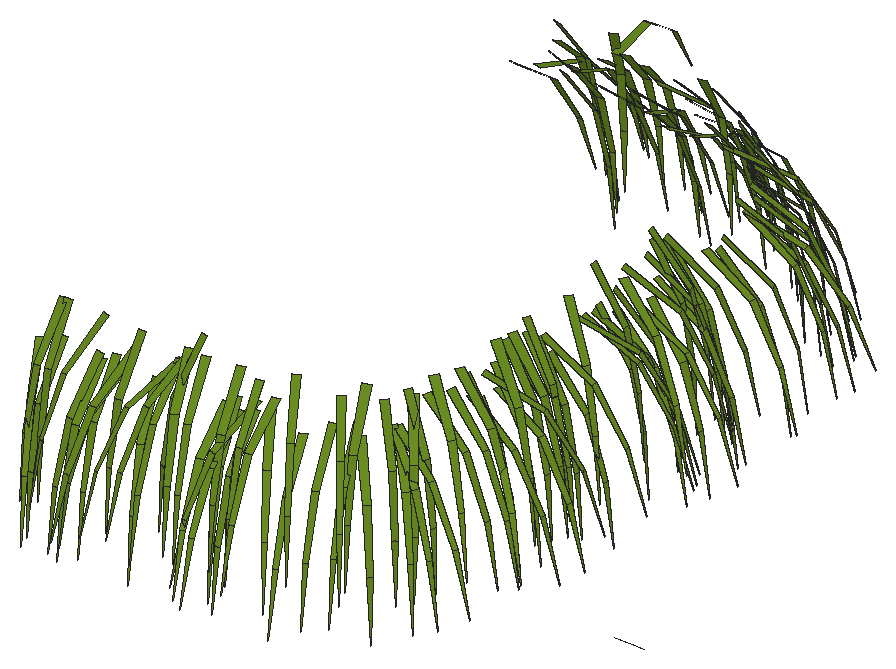
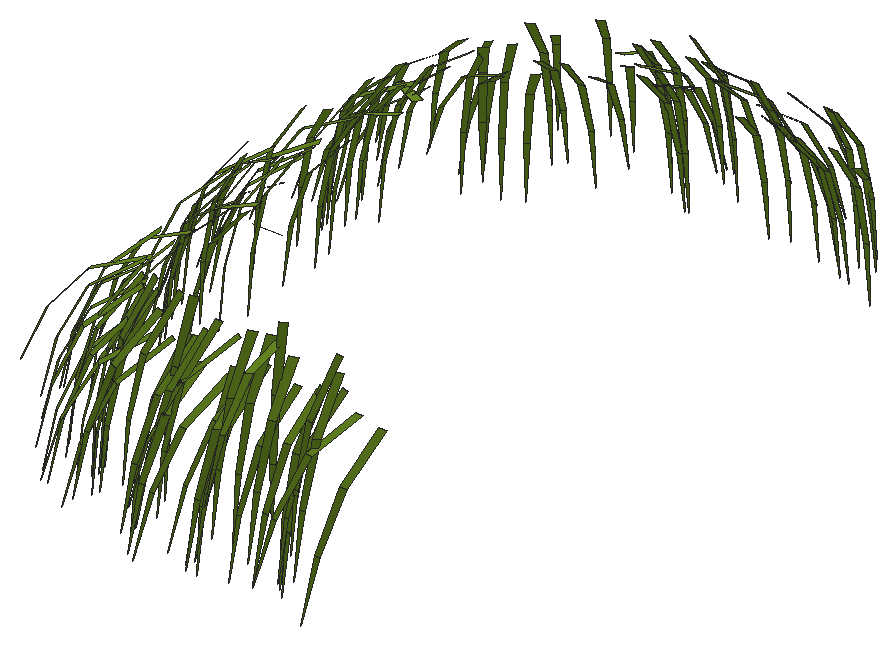
# SketchUp Ruby script. Lengths in inches.
U = 1.inch
M = Sketchup.active_model
def pt(a) = Geom::Point3d.new(a.map { |v| v * U })
def face(e, loops, mat)
  f = e.add_face(loops[0].map { |a| pt(a) })
  loops[1..].each { |l| e.add_face(l.map { |a| pt(a) }).erase! }
  f.material = f.back_material = mat if mat
  f
end
# faces: each face lists its corners as indices into pts; further lists are holes
def faces(e, pts, list, mat = nil) = list.each { |f| face(e, (f[0].is_a?(Array) ? f : [f]).map { |l| l.map { |i| pts[i] } }, mat) }
# xy, xz, yz: faces in a plane at the given z, y or x. An outline is a flat list of corners, or four numbers for a rectangle; further outlines are holes
def ring(l) = l.size == 4 ? [[l[0], l[1]], [l[2], l[1]], [l[2], l[3]], [l[0], l[3]]] : l.each_slice(2).to_a
def flat(e, list, mat, &to3) = list.each { |f| face(e, (f[0].is_a?(Array) ? f : [f]).map { |l| ring(l).map { |u, v| to3.(u, v) } }, mat) }
def xy(e, z, list, mat = nil) = flat(e, list, mat) { |x, y| [x, y, z] }
def xz(e, y, list, mat = nil) = flat(e, list, mat) { |x, z| [x, y, z] }
def yz(e, x, list, mat = nil) = flat(e, list, mat) { |y, z| [x, y, z] }
def lines(e, pts, list) = list.each { |a, b| e.add_line(pt(pts[a]), pt(pts[b])) }
# prism: a flat outline (further loops are holes) pulled along v
def prism(e, loops, v, mat = nil)
  f = face(e, loops, mat); d = Geom::Vector3d.new(v.map { |x| x * U })
  f.pushpull(f.normal.samedirection?(d) ? d.length : -d.length)
end
def box(e, o, s, mat = nil) = prism(e, [[o, [o[0] + s[0], o[1], o[2]], [o[0] + s[0], o[1] + s[1], o[2]], [o[0], o[1] + s[1], o[2]]]], [0, 0, s[2]], mat)
def at(x, y, z, deg = 0) = Geom::Transformation.translation(pt([x, y, z])) * Geom::Transformation.rotation(ORIGIN, Z_AXIS, deg.degrees)
def axes(o, x, y, z) = Geom::Transformation.new([*x, 0, *y, 0, *z, 0, *pt(o).to_a, 1])
def part(name) = M.definitions.add(name)
# library, detail: a bought-in or finely detailed component or shape, given as its bounding box
def library(name, o, s) = part(name).tap { |d| box(d.entities, o, s) }
def detail(e, o, s) = box(e.add_group.entities, o, s)
def put(e, d, t, mat = nil) = e.add_instance(d, t).tap { |i| i.material = mat if mat }
def group(e, t, mat = nil) = e.add_group.tap { |g| g.transformation = t; g.material = mat if mat }.entities
root = M.entities
M.materials.add("[0061_OliveDrab]").color = [107, 142, 35]
p = [[578.37,21.67,546.63],[578.33,21.46,546.63],[578.81,21.49,544.05],[575.9,5.78,546.69],[575.76,5.64,546.69],[576.08,5.46,544.09],
  [563.7,3.375,546.84],[563.51,3.36,546.84],[563.63,3,544.24],[561.71,4.01,546.8],[561.5,4.01,546.8],[561.6,3.83,544.18],
  [575.32,31.82,546.84],[575.47,31.67,546.84],[575.58,31.91,544.23],[563.21,3.55,546.9],[563,3.56,546.9],[563.08,3.2,544.3],
  [578.12,26.57,546.86],[578.17,26.37,546.86],[578.49,26.56,544.26],[574.38,32.14,546.9],[574.5625,32,546.9],[574.6,32.24,544.29],
  [578.36,16.1875,546.95],[578.35,15.98,546.95],[578.74,16.07,544.35],[576.49,31.86,546.99],[576.61,31.7,546.99],[576.97,32.09,544.42],
  [570.74,3.47,547.125],[570.52,3.4375,547.125],[570.68,3.08,544.53],[564.15,33.94,547.14],[564.36,33.9,547.14],[564.31,34.16,544.53],
  [566.98,3.28,547.16],[566.81,3.21,547.16],[567.07,2.8,544.58],[564.56,3.45,547.21],[564.375,3.42,547.21],[564.53,3.08,544.61],
  [562.19,3.09,547.22],[562.02,3,547.22],[562.43,2.45,544.68],[570.31,3.66,547.34],[570.13,3.61,547.34],[570.31,3.32,544.74],
  [574.0625,4.38,547.24],[573.88,4.32,547.24],[574.13,3.89,544.66],[577.73,19.19,547.37],[577.74,19,547.37],[577.94,19.11,544.75],
  [574.89,31.62,547.31],[575.04,31.49,547.31],[575.0625,31.67,544.69],[563.94,3.36,547.4],[563.73,3.44,547.4],[563.7,3.03,544.81],
  [578.58,22.99,547.34],[578.57,22.8,547.34],[579,22.875,544.75],[578.09,27.49,547.37],[578.17,27.33,547.37],[578.46,27.58,544.77],
  [567.45,34.65,547.39],[567.65,34.7,547.39],[567.41,35.2,544.82],[573.63,3.17,547.36],[573.45,3.1,547.36],[573.85,2.36,544.87],
  [577.32,6.34,547.47],[577.19,6.21,547.47],[577.78,5.77,544.95],[577.66,7.01,547.46],[577.57,6.84,547.46],[578.28,6.5625,544.95],
  [575.86,7.28,547.55],[575.74,7.12,547.55],[575.93,7.1,544.93],[577.81,15.24,547.53],[577.78,15.06,547.53],[578.05,15.11,544.92],
  [578.24,29.64,547.43],[578.3125,29.44,547.43],[578.88,29.75,544.88],[567.9,34.46,547.4375],[568.1,34.4,547.4375],[568.14,34.88,544.85],
  [577.52,20.99,547.63],[577.62,20.81,547.63],[577.76,21,545.01],[575.26,33.02,547.54],[575.43,32.92,547.54],[575.63,33.46,544.98],
  [564.09,34.14,547.63],[564.32,34.15,547.63],[564.2,34.41,545.02],[570.8125,34.21,547.625],[571,34.19,547.625],[570.95,34.57,545.03],
  [579.09,19.34,547.66],[579.05,19.14,547.66],[579.67,19.1,545.1],[575.26,4.5,547.75],[575.08,4.42,547.75],[575.43,3.86,545.21],
  [577.83,11.5,547.78],[577.82,11.3,547.78],[578.1,11.38,545.17],[577.7,14.51,547.85],[577.74,14.32,547.85],[577.92,14.45,545.24],
  [575.74,31.7,547.84],[575.9,31.59,547.84],[576.02,31.94,545.24],[565.59,34.92,547.77],[565.79,34.9,547.77],[565.73,35.46,545.2],
  [561.64,35.36,547.65],[561.86,35.35,547.65],[561.79,36.22,545.18],[576.77,8.31,547.92],[576.69,8.14,547.92],[576.91,8.15,545.3],
  [578.61,28.35,547.9],[578.625,28.15,547.9],[579.21,28.29,545.34],[573.31,34.41,547.79],[573.49,34.28,547.79],[573.8125,34.93,545.26],
  [569.02,35.63,547.78],[569.24,35.6,547.78],[569.28,36.52,545.33],[570.52,2.28,547.92],[570.3,2.23,547.92],[570.59,1.39,545.44],
  [576.71,7.35,547.96],[576.54,7.2,547.96],[576.82,7.03,545.35],[579.18,11.57,547.84],[579.17,11.35,547.84],[580.01,11.41,545.35],
  [578.29,12.25,547.97],[578.23,12.08,547.97],[578.64,12.03,545.37],[579.65,21.11,547.87],[579.64,20.91,547.87],[580.54,20.95,545.4],
  [579.08,22.53,547.91],[579.09,22.33,547.91],[579.6875,22.45,545.36],[578.15,23.3125,548.04],[578.15,23.12,548.04],[578.44,23.22,545.43],
  [563.91,34.34,547.98],[564.09,34.28,547.98],[564.1,34.66,545.38],[570.89,3.92,548.1],[570.7,3.89,548.1],[570.83,3.64,545.49],
  [578.78,19.9,548],[578.86,19.6875,548],[579.43,20,545.46],[570.08,2.31,548.11],[569.875,2.26,548.11],[570.17,1.48,545.62],
  [565.27,4.08,548.2],[565.07,4.09,548.2],[565.17,3.88,545.59],[578.47,7.47,548.01],[578.4,7.29,548.01],[579.38,7.04,545.58],
  [578.68,10.18,548.12],[578.63,9.98,548.12],[579.32,9.93,545.58],[579.62,12.55,548.09],[579.58,12.36,548.09],[580.42,12.3,545.6],
  [573.73,32.59,548.22],[573.87,32.45,548.22],[573.93,32.65,545.6],[572.96,33.31,548.16],[573.17,33.28,548.16],[573.11,33.63,545.55],
  [574.61,33.96,548.15],[574.75,33.81,548.15],[575.21,34.37,545.63],[567.05,34.93,548.14],[567.27,34.91,548.14],[567.22,35.54,545.59],
  [562.05,4.16,548.31],[561.86,4.15,548.31],[561.97,3.99,545.6875],[579.46,24.91,548.23],[579.4375,24.71,548.23],[580.21,24.74,545.71],
  [576.26,32.43,548.31],[576.41,32.27,548.31],[576.75,32.74,545.75],[567.98,35.06,548.2],[568.16,35,548.2],[568.29,35.77,545.69],
  [569.32,35.82,548.16],[569.54,35.84,548.16],[569.33,36.75,545.7],[567.51,2.91,548.36],[567.32,2.88,548.36],[567.51,2.32,545.8],
  [573.11,3.19,548.27],[572.96,3.09,548.27],[573.48,2.5,545.76],[577.97,13.37,548.37],[577.92,13.15,548.37],[578.21,13.2,545.76],
  [578.27,14.2,548.39],[578.22,14.02,548.39],[578.59,14.01,545.79],[579.15,19.0625,548.3],[579.2,18.88,548.3],[579.95,19.15,545.8],
  [575.64,31.8,548.43],[575.78,31.65,548.43],[575.91,31.92,545.82],[566.9,35.66,548.29],[567.11,35.7,548.29],[566.85,36.51,545.8],
  [564.56,2.5,548.36],[564.35,2.53,548.36],[564.35,1.73,545.86],[570.03,2.42,548.46],[569.85,2.45,548.46],[569.84,1.71,545.9375],
  [571.31,3.41,548.51],[571.14,3.37,548.51],[571.33,3.02,545.91],[561.71,3.7,548.5],[561.51,3.69,548.5],[561.62,3.42,545.89],
  [574.98,5.66,548.54],[574.79,5.58,548.54],[574.99,5.36,545.93],[578.58,9.14,548.5],[578.54,8.93,548.5],[579.16,8.92,545.94],
  [577.43,22.4,548.54],[577.45,22.2,548.54],[577.59,22.3125,545.92],[572.93,34.5,548.42],[573.13,34.45,548.42],[573.2,35.09,545.875],
  [570.125,35.26,548.46],[570.32,35.25,548.46],[570.25,35.99,545.9375],[570.39,3.61,548.66],[570.1875,3.57,548.66],[570.35,3.31,546.05],
  [578.23,22.79,548.57],[578.23,22.56,548.57],[578.55,22.67,545.97],[577.96,28.93,548.6],[578.07,28.75,548.6],[578.41,29.09,546.02],
  [578.01,30.03,548.58],[578.08,29.83,548.58],[578.61,30.13,546.03],[573.41,32.63,548.62],[573.61,32.51,548.62],[573.6,32.71,546],
  [569.04,3.31,548.73],[568.85,3.25,548.73],[569.07,2.87,546.14],[577.95,16.15,548.68],[577.85,15.97,548.68],[578.25,15.87,546.09],
  [578.33,22.85,548.68],[578.4,22.67,548.68],[578.77,22.92,546.09],[569.76,34.97,548.62],[569.96,34.95,548.62],[569.91,35.54,546.06],
  [565.72,2.7,548.78],[565.54,2.78,548.78],[565.375,2.14,546.24],[562.74,3.28,548.8],[562.5625,3.34,548.8],[562.49,2.85,546.22],
  [578.14,12.17,548.8],[578.06,11.97,548.8],[578.4375,11.93,546.2],[578.01,14.3,548.82],[577.96,14.11,548.82],[578.27,14.125,546.21],
  [578.59,13.33,548.93],[578.53,13.125,548.93],[579,13.1,546.34],[579.14,19.37,548.77],[579.22,19.19,548.77],[579.89,19.59,546.26],
  [569.35,34.52,548.91],[569.54,34.5,548.91],[569.5,34.87,546.31],[575.52,4.5,548.88],[575.37,4.39,548.88],[575.93,3.8125,546.38],
  [567.64,4.12,549.06],[567.46,4.17,549.06],[567.51,3.98,546.44],[579.41,13.61,548.92],[579.47,13.39,548.92],[580.22,13.73,546.42],
  [579.5625,15.9375,548.86],[579.5625,15.74,548.86],[580.47,15.84,546.39],[569.88,33.62,549],[570.09,33.65,549],[569.96,33.82,546.38],
  [571.67,33.71,549],[571.875,33.63,549],[571.86,33.89,546.39],[563.69,35.75,548.875],[563.89,35.78,548.875],[563.65,36.68,546.42],
  [572.18,2.46,548.99],[571.99,2.41,548.99],[572.29,1.61,546.51],[568.72,3.1,549.07],[568.52,3.01,549.07],[568.83,2.56,546.5],
  [578.11,8.28,549.05],[577.99,8.1,549.05],[578.55,7.86,546.5],[578.85,10.14,549.07],[578.78,9.93,549.07],[579.43,9.82,546.53],
  [577.68,18.96,549.14],[577.7,18.75,549.14],[577.91,18.87,546.52],[578.5625,23.92,549.04],[578.63,23.7,549.04],[579.14,23.99,546.48],
  [579.31,28.97,548.93],[579.36,28.76,548.93],[580.36,29.125,546.53],[563.68,34.04,549.12],[563.875,34.02,549.12],[563.8125,34.31,546.51],
  [566.75,34.62,549.11],[566.96,34.67,549.11],[566.74,35.15,546.54],[562.61,34.97,549.04],[562.8,35.02,549.04],[562.52,35.73,546.52],
  [566.89,2.65,549.17],[566.7,2.6875,549.17],[566.66,2.01,546.63],[579.37,9.61,548.89],[579.25,9.44,548.89],[580.29,8.81,546.56],
  [579.22,19.2,549.07],[579.15,19,549.07],[579.9,18.83,546.56],[577.46,21.86,549.09],[577.41,21.56,549.09],[577.93,22.57,549.25],
  [577.97,22.39,549.25],[578.22,22.54,546.64],[565.9,34.52,549.17],[566.12,34.57,549.17],[565.9,35.03,546.59],[569.97,34.78,549.17],
  [570.13,34.68,549.17],[570.43,35.3125,546.63],[563.06,36.09,548.99],[563.26,36.0625,548.99],[563.3,37.11,546.58],[573.62,3.9,549.21],
  [573.45,3.8,549.21],[573.85,3.36,546.66],[575.33,6.4,549.18],[575.13,6.2,549.18],[578.93,21.66,549.22],[579.01,21.45,549.22],
  [579.59,21.77,546.68],[565.3,33.29,549.29],[565.49,33.38,549.29],[565.32,33.48,546.67],[564.55,35.14,549.18],[564.77,35.2,549.18],
  [564.43,35.96,546.68],[563.66,4.2,549.33],[563.39,4.18,549.33],[561.74,4.54,549.37],[561.45,4.53,549.37],[574.84,31.41,549.39],
  [575.04,31.19,549.39],[563.3,4.32,549.41],[563.01,4.34,549.41],[577.5,16.26,549.43],[577.49,15.98,549.43],[577.33,26.42,549.36],
  [577.41,26.14,549.36],[574.02,31.73,549.47],[574.28,31.54,549.47],[575.62,31.26,549.4],[575.79,31.02,549.4],[570.68,4.31,549.61],
  [570.37,4.27,549.61],[563.98,33.35,549.6875],[564.27,33.28,549.6875],[561.64,4.19,549.53],[561.4,4.06,549.53],[566.67,4.22,549.59],
  [566.42,4.12,549.59],[564.44,4.27,549.71],[564.1875,4.22,549.71],[573.79,5.32,549.67],[573.53,5.24,549.67],[570.15,4.39,549.86],
  [569.9,4.32,549.86],[577.64,23.07,549.8],[577.63,22.8,549.8],[574.55,31.3125,549.9],[574.76,31.12,549.9],[573.14,4.49,549.57],
  [572.88,4.39,549.57],[564.27,4.17,549.875],[563.97,4.28,549.875],[577.17,19.2,549.93],[577.1875,18.93,549.93],[577.29,27.14,549.84],
  [577.41,26.9,549.84],[577.08,29.28,549.75],[577.18,29,549.75],[567.58,33.58,549.89],[567.88,33.49,549.89],[567.68,33.62,549.79],
  [567.96,33.69,549.79],[576.39,7.29,549.73],[576.21,7.1,549.73],[576.52,7.68,549.73],[576.39,7.44,549.73],[577.18,15.375,550.08],
  [577.14,15.12,550.08],[574.66,32.08,549.92],[574.9,31.9375,549.92],[575.53,7.6,550.14],[575.35,7.39,550.14],[576.98,20.75,550.1875],
  [577.11,20.5,550.1875],[570.67,33.4,550.12],[570.9375,33.37,550.12],[564.0625,33.47,550.17],[564.38,33.48,550.17],[574.8125,5.66,550.0625],
  [574.56,5.55,550.0625],[577.9,19.66,549.97],[577.84,19.39,549.97],[561.52,33.96,549.87],[561.83,33.94,549.87],[577.17,11.57,550.32],
  [577.16,11.3,550.32],[577.81,11.7,550.07],[577.79,11.39,550.07],[575.24,31.0625,550.34],[575.47,30.9,550.34],[572.53,33.37,550.07],
  [572.78,33.19,550.07],[565.47,33.84,550.16],[565.74,33.8125,550.16],[568.74,34.13,549.92],[569.05,34.08,549.92],[570.25,3.75,550.07],
  [569.95,3.68,550.07],[576.29,8.57,550.49],[576.18,8.33,550.49],[577.14,14.43,550.42],[577.19,14.16,550.42],[578.1,21.25,549.98],
  [578.08,20.97,549.98],[577.875,22.53,550.25],[577.88,22.25,550.25],[577.43,28.3,550.24],[577.45,28.02,550.24],[576.26,7.96,550.47],
  [576.01,7.76,550.47],[576.96,8.05,550.07],[576.87,7.8,550.07],[577.47,12.57,550.4375],[577.38,12.33,550.4375],[577.62,19.55,550.33],
  [577.73,19.25,550.33],[577.42,23.35,550.5625],[577.42,23.08,550.5625],[563.64,33.56,550.48],[563.89,33.48,550.48],[569.79,3.74,550.29],
  [569.5,3.67,550.29],[570.83,4.57,550.65],[570.57,4.53,550.65],[577.5,10.48,550.45],[577.4375,10.2,550.45],[578.125,12.87,550.22],
  [578.07,12.59,550.22],[566.89,33.8,550.5],[567.21,33.77,550.5],[565.32,4.61,550.77],[565.03,4.61,550.77],[578.05,25.07,550.4375],
  [578.03,24.79,550.4375],[573.33,32.26,550.79],[573.53,32.0625,550.79],[572.82,32.5625,550.67],[573.11,32.52,550.67],[573.58,33.07,550.4],
  [573.78,32.85,550.4],[567.57,33.82,550.48],[567.8125,33.75,550.48],[569.43,34.22,550.24],[569.74,34.25,550.24],[572.35,4.375,550.48],
  [572.125,4.22,550.48],[562.06,4.63,550.89],[561.79,4.61,550.89],[577.81,18.79,550.54],[577.87,18.53,550.54],[575.4,31.6875,550.67],
  [575.61,31.46,550.67],[567.14,34.16,550.43],[567.43,34.22,550.43],[564.77,3.84,550.62],[564.47,3.875,550.62],[567.375,4.02,550.74],
  [567.1,3.98,550.74],[577.31,13.54,550.9],[577.25,13.23,550.9],[577.48,14.47,550.88],[577.41,14.21,550.88],[575.1,31.34,550.96],
  [575.3,31.14,550.96],[572.56,33.37,550.76],[572.85,33.29,550.76],[570.25,3.78,550.7],[570,3.8125,550.7],[571.12,4.28,550.98],
  [570.87,4.21,550.98],[561.74,4.375,551.04],[561.46,4.37,551.04],[574.77,6.3125,551.07],[574.5,6.2,551.07],[577.42,9.41,550.84],
  [577.36,9.12,550.84],[576.97,22.39,551.12],[577,22.11,551.12],[570.03,33.95,550.73],[570.3125,33.94,550.73],[577.47,22.84,551.08],
  [577.47,22.52,551.08],[577.08,28.42,551.02],[577.24,28.17,551.02],[576.87,29.67,550.92],[576.97,29.39,550.92],[573.125,32.26,551.2],
  [573.4,32.09,551.2],[569.63,33.85,550.99],[569.92,33.83,550.99],[568.81,4.21,551.18],[568.54,4.13,551.18],[570.27,4.33,551.18],
  [569.98,4.26,551.18],[577.23,16.58,551.17],[577.1,16.33,551.17],[577.44,22.55,551.13],[577.54,22.3,551.13],[566.25,3.86,551.08],
  [566,3.96,551.08],[563.09,4.19,551.24],[562.84,4.28,551.24],[577.4,12.54,551.29],[577.28,12.25,551.29],[577.33,14.53,551.34],
  [577.26,14.27,551.34],[577.81,18.83,550.97],[577.92,18.57,550.97],[574.72,5.6,551.125],[574.52,5.44,551.125],[577.86,10.76,550.7],
  [577.69,10.52,550.7],[577.96,13.24,551.08],[578.05,12.9375,551.08],[577.66,13.65,551.36],[577.57,13.36,551.36],[578.03,15.97,550.99],
  [578.03,15.69,550.99],[577.65,28.61,550.93],[577.72,28.3125,550.93],[569.19,33.6875,551.4],[569.46,33.65,551.4],[563.9,34.18,550.97],
  [564.18,34.22,550.97],[571.85,3.9375,551.13],[571.57,3.87,551.13],[577.51,23.62,551.43],[577.61,23.32,551.43],[571.4,33.13,551.55],
  [571.69,33.02,551.55],[569.92,33.11,551.57],[570.2,33.15,551.57],[562.89,33.73,551.33],[563.16,33.81,551.33],[562.8,34.35,550.94],
  [563.08,34.32,550.94],[568.33,4.125,551.46],[568.04,4,551.46],[567.81,4.59,551.64],[567.55,4.66,551.64],[577.17,8.96,551.4],
  [577,8.71,551.4],[577.69,10.6,551.38],[577.59,10.31,551.38],[577.11,18.96,551.7],[577.13,18.66,551.7],[577.92,19.73,551.28],
  [577.82,19.46,551.28],[575.74,22.17,551.04],[575.68,21.8,551.04],[563.5625,33.38,551.66],[563.84,33.35,551.66],[566.95,33.61,551.53],
  [567.24,33.68,551.53],[567.18,3.86,551.48],[566.92,3.91,551.48],[573.0625,4.84,551.6],[572.83,4.7,551.6],[574.03,7.74,551.03],
  [573.79,7.49,551.03],[577.73,21.3,551.53],[577.83,21,551.53],[566.08,33.5625,551.61],[566.38,33.63,551.61],[569.24,33.72,551.45],
  [569.46,33.58,551.45],[564.89,33.81,551.42],[565.19,33.9,551.42],[563.54,5.97,551.26],[563.2,5.94,551.26],[577.26,22.47,551.79],
  [577.3125,22.21,551.79],[565.46,32.87,551.875],[565.72,32.99,551.875],[563.44,5.95,551.47],[563.08,5.97,551.47],[561.76,5.96,551.57],
  [561.4,5.96,551.57],[575.71,16.37,551.35],[575.7,16.02,551.35],[575.66,26.05,551.35],[575.75,25.7,551.35],[574.01,30.08,551.1],
  [574.22,29.79,551.1],[573.7,30.36,551.51],[573.96,30.1,551.51],[560.67,6.04,551.125],[560.38,5.88,551.125],[573.18,30.67,551.72],
  [573.49,30.44,551.72],[566.01,6.02,551.38],[565.71,5.9,551.38],[570.49,6.07,551.54],[570.1,6.02,551.54],[572.34,6.53,551.03],
  [572.04,6.4,551.03],[564.16,5.99,551.66],[563.84,5.93,551.66],[573.22,7.1,551.52],[572.91,7,551.52],[574.81,8.84,551.14],
  [574.59,8.61,551.14],[574.67,8.72,551.28],[574.52,8.43,551.28],[563.62,31.87,551.83],[563.97,31.79,551.83],[575.71,23.1875,551.57],
  [575.7,22.86,551.57],[575.6,26.32,551.67],[575.74,26.03,551.67],[575.05,28.61,551.28],[575.18,28.27,551.28],[568.14,31.78,551.61],
  [568.48,31.875,551.61],[565.07,36.49,551.93],[565.28,36.53,551.93],[564.85,37.94,549.76],[564.91,5.9,551.75],[564.55,6.02,551.75],
  [569.74,6,551.89],[569.43,5.92,551.89],[575.7,19.16,552.1],[575.71,18.82,552.1],[573.66,30.375,552.18],[573.92,30.14,552.18],
  [573.61,30.36,551.6],[573.91,30.1875,551.6],[561.375,31.84,551.41],[561.76,31.82,551.41],[567.04,31.88,551.82],[567.4,31.77,551.82],
  [568.35,31.86,551.17],[568.73,31.8,551.17],[575.75,20.21,551.36],[575.67,19.88,551.36],[575.72,21.43,551.07],[575.7,21.09,551.07],
  [569.81,6,551.34],[569.43,5.92,551.34],[574,7.63,551.58],[573.68,7.5,551.58],[574.53,8.45,552.41],[574.32,8.1875,552.41],
  [574.75,8.875,551.24],[574.64,8.57,551.24],[575.69,11.86,551.61],[575.67,11.47,551.61],[575.73,15.63,552.25],[575.68,15.32,552.25],
  [571.27,31.625,551.57],[571.57,31.41,551.57],[570.44,31.7,552.1],[570.76,31.66,552.1],[575.74,13.35,551.2],[575.67,13.01,551.2],
  [575.62,20.08,552.33],[575.79,19.76,552.33],[575.7,22.49,551.72],[575.71,22.15,551.72],[575.29,28.18,551.76],[575.32,27.84,551.76],
  [564.07,31.82,552.21],[564.46,31.83,552.21],[565.27,31.84,551.85],[565.61,31.81,551.85],[569.64,31.81,551.26],[570.02,31.85,551.26],
  [569.29,6,551.52],[568.93,5.92,551.52],[575.66,11.6875,552.47],[575.64,11.35,552.47],[575.64,18.91,551.93],[575.77,18.54,551.93],
  [574.22,29.67,552.32],[574.5,29.47,552.32],[575.54,10.95,552.13],[575.46,10.6,552.13],[575.76,13.19,552.33],[575.65,12.89,552.33],
  [575.67,14.16,552.58],[575.74,13.82,552.58],[575.72,25.3,551.625],[575.69,24.96,551.625],[571.87,31.54,551.67],[572.12,31.27,551.67],
  [567.55,31.79,551.49],[567.9,31.86,551.49],[571.08,6.27,551.78],[570.81,6.08,551.78],[575.17,9.34,552.43],[574.875,9.09,552.43],
  [574.98,9.1875,552.67],[574.84,8.9,552.67],[575.67,18.31,551.99],[575.74,18,551.99],[563.1,31.875,552.42],[563.42,31.78,552.42],
  [566.66,31.85,552.24],[567.05,31.81,552.24],[566.94,31.875,552.12],[567.24,31.78,552.12],[565.07,5.9375,552.16],[564.71,5.98,552.16],
  [570.64,6.11,552.77],[570.3125,6.06,552.77],[575.71,23.38,552.55],[575.71,23.05,552.55],[570.6,6.05,551.95],[570.29,6.1,551.95],
  [567.09,5.99,552.45],[566.76,5.93,552.45],[575.8125,12.28,551.3],[575.6,11.99,551.3],[573.84,30.27,552.24],[574.1,30,552.24],
  [572.57,30.97,552.74],[572.93,30.92,552.74],[569.91,31.79,552.22],[570.26,31.78,552.22],[565.37,5.96,553.03],[565.02,5.96,553.03],
  [575.32,9.86,552.34],[575.25,9.49,552.34],[572.3,31.29,553.01],[572.54,31.05,553.01],[571.97,31.4,552.39],[572.32,31.3,552.39],
  [561.99,5.97,553.15],[561.66,5.95,553.15],[575.74,13.89,552.98],[575.67,13.51,552.98],[575.75,15.01,552.78],[575.66,14.69,552.78],
  [575.28,28.0625,551.9375],[575.375,27.7,551.9375],[574.82,28.96,552.39],[574.94,28.62,552.39],[562.44,31.85,551.65],[562.79,31.81,551.65],
  [570.65,6.13,552.79],[570.34,6.04,552.79],[561.75,5.96,553.13],[561.41,5.96,553.13],[575.71,15.99,552.2],[575.71,15.65,552.2],
  [575.64,17.91,552.11],[575.78,17.59,552.11],[575.37,27.35,552.7],[575.5625,27.05,552.7],[573.89,30.22,553],[574.125,29.97,553],
  [564.23,31.8,552.03],[564.58,31.86,552.03],[569.44,31.84,552.67],[569.79,31.81,552.67],[567.14,5.89,552.47],[566.83,6.02,552.47],
  [571.3,6.25,552.23],[570.96,6.17,552.23],[573.44,7.32,552.65],[573.19,7.12,552.65],[574.22,7.82,553.15],[573.88,7.69,553.15],
  [575.65,12.61,552.16],[575.76,12.24,552.16],[575.65,21.89,552.93],[575.77,21.58,552.93],[575.6875,22.29,553.41],[575.72,21.95,553.41],
  [575.71,22.88,553.03],[575.71,22.48,553.03],[568.3,6.01,553.02],[567.98,5.91,553.02],[563.71,5.91,553.125],[563.4,6.01,553.125],
  [569.91,6,553.17],[569.5625,5.92,553.17],[575.79,17.41,553.2],[575.62,17.1,553.2],[572.4,31.17,553.48],[572.74,30.96,553.48],
  [575.78,13.27,553.22],[575.63,12.92,553.22],[575.75,15.01,553.38],[575.66,14.6875,553.38],[575.77,20.58,552.53],[575.64,20.24,552.53],
  [563.37,31.78,553.02],[563.7,31.87,553.02],[575.45,10.15,553],[575.24,9.84,553],[575.65,11.36,552.84],[575.52,11.01,552.84],
  [575.76,14.25,553.07],[575.65,13.88,553.07],[575.65,23.05,553.1875],[575.77,22.68,553.1875],[565.44,31.77,552.97],[565.82,31.88,552.97],
  [568.9,31.85,553.25],[569.23,31.81,553.25],[567.64,5.93,553.03],[567.3125,5.99,553.03],[567.55,6.04,553.08],[567.2,5.88,553.08],
  [575.64,20.63,552.98],[575.77,20.26,552.98],[570.81,31.67,553.65],[571.17,31.54,553.65],[568.02,31.92,552.92],[568.3,31.74,552.92],
  [567.34,31.79,553.37],[567.7,31.87,553.37],[568.19,5.92,553.87],[567.88,6,553.87],[572.0625,6.46,553.41],[571.78,6.28,553.41],
  [570.09,31.72,553.79],[570.44,31.77,553.79],[566.45,31.79,553.5],[566.83,31.87,553.5],[566.43,31.88,553.4],[575.69,18.88,553.91],
  [575.72,18.52,553.91],[563.35,31.85,553.77],[563.69,31.81,553.77],[575.67,22.17,553.86],[575.74,21.86,553.86],[565.96,31.75,554.2],
  [566.28,31.91,554.2],[565.52,34.35,553.39],[565.8125,34.42,553.39],[566.08,31.79,553.4],[566.4375,31.87,553.4],[581.95,12.12,543.57],
  [583.33,12.12,543.57]]
faces(root,p,[[0,1,2],[3,4,5],[6,7,8],[9,10,11],[12,13,14],[15,16,17],[18,19,20],[21,22,23],
  [24,25,26],[27,28,29],[30,31,32],[33,34,35],[36,37,38],[39,40,41],[42,43,44],[45,46,47],
  [48,49,50],[51,52,53],[54,55,56],[57,58,59],[60,61,62],[63,64,65],[66,67,68],[69,70,71],
  [72,73,74],[75,76,77],[78,79,80],[81,82,83],[84,85,86],[87,88,89],[90,91,92],[93,94,95],
  [96,97,98],[99,100,101],[102,103,104],[105,106,107],[108,109,110],[111,112,113],[114,115,116],[117,118,119],
  [120,121,122],[123,124,125],[126,127,128],[129,130,131],[132,133,134],[135,136,137],[138,139,140],[141,142,143],
  [144,145,146],[147,148,149],[150,151,152],[153,154,155],[156,157,158],[159,160,161],[162,163,164],[165,166,167],
  [168,169,170],[171,172,173],[174,175,176],[177,178,179],[180,181,182],[183,184,185],[186,187,188],[189,190,191],
  [192,193,194],[195,196,197],[198,199,200],[201,202,203],[204,205,206],[207,208,209],[210,211,212],[213,214,215],
  [216,217,218],[219,220,221],[222,223,224],[225,226,227],[228,229,230],[231,232,233],[234,235,236],[237,238,239],
  [240,241,242],[243,244,245],[246,247,248],[249,250,251],[252,253,254],[255,256,257],[258,259,260],[261,262,263],
  [264,265,266],[267,268,269],[270,271,272],[273,274,275],[276,277,278],[279,280,281],[282,283,284],[285,286,287],
  [288,289,290],[291,292,293],[294,295,296],[297,298,299],[300,301,302],[303,304,305],[306,307,308],[309,310,311],
  [312,313,314],[315,316,317],[318,319,320],[321,322,323],[324,325,326],[327,328,329],[330,331,332],[333,334,335],
  [336,337,338],[339,340,341],[342,343,344],[345,346,347],[348,349,350],[351,352,353],[354,355,356],[357,358,359],
  [360,361,362],[363,364,1,0],[365,366,367],[368,369,370],[371,372,373],[374,375,376],[377,378,379],[380,381,4,3],
  [382,383,384],[385,386,387],[388,389,390],[391,392,7,6],[393,394,10,9],[395,396,13,12],[397,398,16,15],[399,400,25,24],
  [401,402,19,18],[403,404,22,21],[405,406,28,27],[407,408,31,30],[409,410,34,33],[411,412,43,42],[413,414,37,36],[415,416,40,39],
  [417,418,49,48],[419,420,46,45],[421,422,61,60],[423,424,55,54],[425,426,70,69],[427,428,58,57],[429,430,52,51],[431,432,64,63],
  [433,434,85,84],[435,436,88,87],[437,438,67,66],[439,440,73,72],[441,442,76,75],[443,444,82,81],[445,446,94,93],[447,448,79,78],
  [449,450,91,90],[451,452,100,99],[453,454,97,96],[455,456,106,105],[457,458,103,102],[459,460,121,120],[461,462,109,108],[463,464,142,141],
  [465,466,115,114],[467,468,130,129],[469,470,118,117],[471,472,133,132],[473,474,136,135],[475,476,124,123],[477,478,112,111],[479,480,148,147],
  [481,482,151,150],[483,484,127,126],[485,486,139,138],[487,488,172,171],[489,490,145,144],[491,492,163,162],[493,494,154,153],[495,496,157,156],
  [497,498,166,165],[499,500,160,159],[501,502,175,174],[503,504,178,177],[505,506,190,189],[507,508,169,168],[509,510,196,195],[511,512,181,180],
  [513,514,184,183],[515,516,187,186],[517,518,202,201],[519,520,205,204],[521,522,211,210],[523,524,193,192],[525,526,220,219],[527,528,199,198],
  [529,530,226,225],[531,532,229,228],[533,534,208,207],[535,536,214,213],[537,538,217,216],[539,540,223,222],[541,542,250,249],[543,544,232,231],
  [545,546,235,234],[547,548,238,237],[549,550,241,240],[551,552,244,243],[553,554,247,246],[555,556,253,252],[557,558,259,258],[559,560,262,261],
  [561,562,265,264],[563,564,268,267],[565,566,280,279],[567,568,271,270],[569,570,256,255],[571,572,274,273],[573,574,277,276],[575,576,283,282],
  [577,578,286,285],[579,580,289,288],[581,582,292,291],[583,584,298,297],[585,586,304,303],[587,588,358,357],[589,590,310,309],[591,592,295,294],
  [593,594,313,312],[595,596,343,342],[597,598,301,300],[599,600,322,321],[601,602,325,324],[603,604,340,339],[605,606,319,318],[607,608,316,315],
  [609,610,352,351],[611,612,375,374],[613,614,328,327],[615,616,307,306],[617,618,331,330],[619,620,334,333],[621,622,337,336],[623,624,361,360],
  [625,626,364,363],[627,628,346,345],[629,630,349,348],[631,632,355,354],[633,634,378,377],[635,636,381,380],[637,638,383,382],[639,640,369,368],
  [641,642,372,371],[643,644,389,388],[645,646,392,391],[647,648,366,365],[649,650,386,385],[651,652,398,397],[653,654,394,393],[655,656,400,399],
  [657,658,402,401],[659,660,406,405],[661,662,396,395],[663,664,412,411],[665,666,404,403],[667,668,414,413],[669,670,408,407],[671,672,426,425],
  [673,674,416,415],[675,676,418,417],[677,678,440,439],[679,680,442,441],[681,682,410,409],[683,684,422,421],[685,686,432,431],[687,688,434,433],
  [689,690,438,437],[691,692,693],[694,695,428,427],[696,697,420,419],[698,699,430,429],[700,701,424,423],[702,703,446,445],[704,705,460,459],
  [706,707,436,435],[708,709,472,471],[710,711,458,457],[712,713,480,479],[714,715,474,473],[716,717,456,455],[718,719,448,447],[720,721,488,487],
  [722,723,464,463],[724,725,444,443],[726,727,468,467],[728,729,452,451],[730,731,504,503],[732,733,450,449],[734,735,482,481],[736,737,484,483],
  [738,739,454,453],[740,741,470,469],[742,743,520,519],[744,745,498,497],[746,747,462,461],[748,749,492,491],[750,751,466,465],[752,753,502,501],
  [754,755,490,489],[756,757,478,477],[758,759,510,509],[760,761,516,515],[762,763,530,529],[764,765,522,521],[766,767,486,485],[768,769,476,475],
  [770,771,526,525],[772,773,496,495],[774,775,506,505],[776,777,518,517],[778,779,532,531],[780,781,500,499],[782,783,494,493],[784,785,544,543],
  [786,787,534,533],[788,789,588,587],[790,791,528,527],[792,793,514,513],[794,795,556,555],[796,797,508,507],[798,799,552,551],[800,801,512,511],
  [802,803,542,541],[804,805,524,523],[806,807,536,535],[808,809,538,537],[810,811,596,595],[812,813,562,561],[814,815,612,611],[816,817,546,545],
  [818,819,548,547],[820,821,594,593],[822,823,584,583],[824,825,560,559],[826,827,540,539],[828,829,600,599],[830,831,566,565],[832,833,576,575],
  [834,835,602,601],[836,837,586,585],[838,839,550,549],[840,841,590,589],[842,843,574,573],[844,845,554,553],[846,847,558,557],[848,849,568,567],
  [850,851,578,577],[852,853,570,569],[854,855,572,571],[856,857,564,563],[858,859,580,579],[860,861,582,581],[862,863,624,623],[864,865,610,609],
  [866,867,618,617],[868,869,620,619],[870,871,592,591],[872,873,604,603],[874,875,644,643],[876,877,598,597],[878,879,632,631],[880,881,614,613],
  [882,883,638,637],[884,885,606,605],[886,887,642,641],[888,889,630,629],[890,891,616,615],[892,893,634,633],[894,895,608,607],[896,897,640,639,898],
  [899,900,622,621],[901,902,628,627],[903,904,648,647],[905,906,650,649],[907,908,692,691],[909,910,898,908,907]],"[0061_OliveDrab]")
lines(root,p,[[911,912]])
